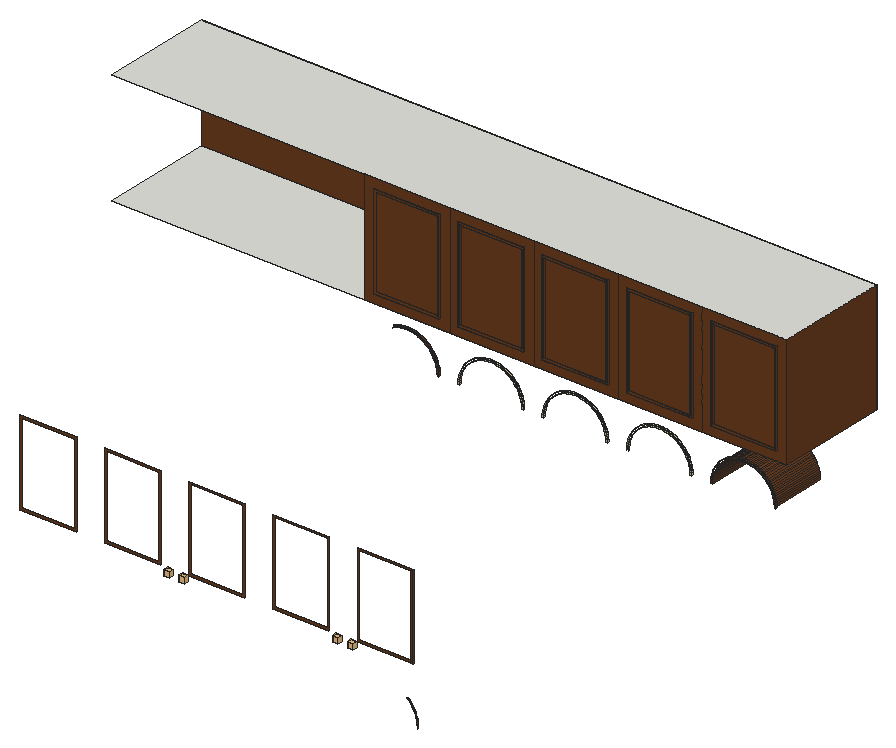
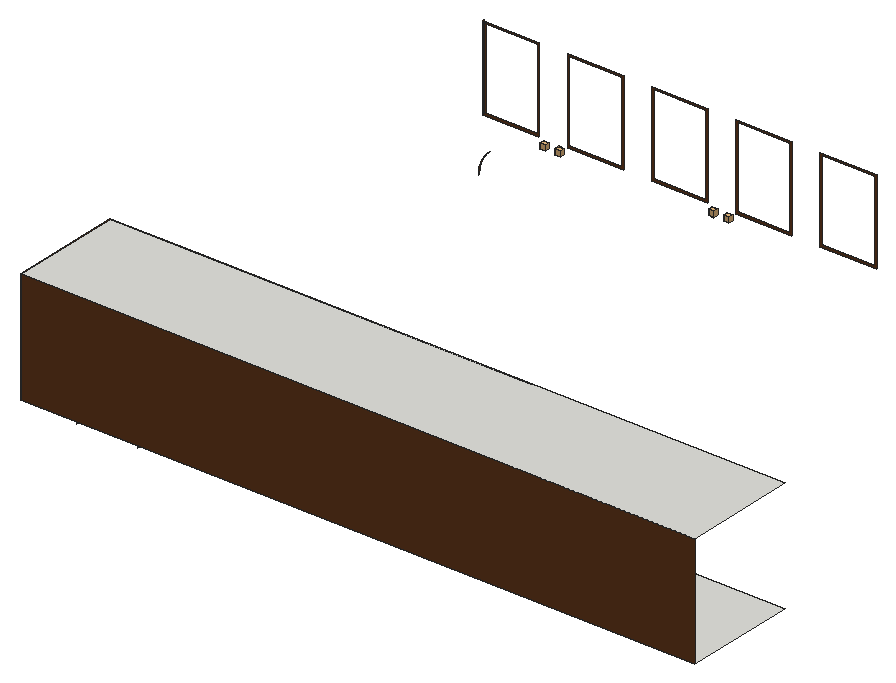
# SketchUp Ruby script. Lengths in inches.
U = 1.inch
M = Sketchup.active_model
def pt(a) = Geom::Point3d.new(a.map { |v| v * U })
def face(e, loops, mat)
  f = e.add_face(loops[0].map { |a| pt(a) })
  loops[1..].each { |l| e.add_face(l.map { |a| pt(a) }).erase! }
  f.material = f.back_material = mat if mat
  f
end
# faces: each face lists its corners as indices into pts; further lists are holes
def faces(e, pts, list, mat = nil) = list.each { |f| face(e, (f[0].is_a?(Array) ? f : [f]).map { |l| l.map { |i| pts[i] } }, mat) }
# xy, xz, yz: faces in a plane at the given z, y or x. An outline is a flat list of corners, or four numbers for a rectangle; further outlines are holes
def ring(l) = l.size == 4 ? [[l[0], l[1]], [l[2], l[1]], [l[2], l[3]], [l[0], l[3]]] : l.each_slice(2).to_a
def flat(e, list, mat, &to3) = list.each { |f| face(e, (f[0].is_a?(Array) ? f : [f]).map { |l| ring(l).map { |u, v| to3.(u, v) } }, mat) }
def xy(e, z, list, mat = nil) = flat(e, list, mat) { |x, y| [x, y, z] }
def xz(e, y, list, mat = nil) = flat(e, list, mat) { |x, z| [x, y, z] }
def yz(e, x, list, mat = nil) = flat(e, list, mat) { |y, z| [x, y, z] }
def lines(e, pts, list) = list.each { |a, b| e.add_line(pt(pts[a]), pt(pts[b])) }
# prism: a flat outline (further loops are holes) pulled along v
def prism(e, loops, v, mat = nil)
  f = face(e, loops, mat); d = Geom::Vector3d.new(v.map { |x| x * U })
  f.pushpull(f.normal.samedirection?(d) ? d.length : -d.length)
end
def box(e, o, s, mat = nil) = prism(e, [[o, [o[0] + s[0], o[1], o[2]], [o[0] + s[0], o[1] + s[1], o[2]], [o[0], o[1] + s[1], o[2]]]], [0, 0, s[2]], mat)
def at(x, y, z, deg = 0) = Geom::Transformation.translation(pt([x, y, z])) * Geom::Transformation.rotation(ORIGIN, Z_AXIS, deg.degrees)
def axes(o, x, y, z) = Geom::Transformation.new([*x, 0, *y, 0, *z, 0, *pt(o).to_a, 1])
def part(name) = M.definitions.add(name)
# library, detail: a bought-in or finely detailed component or shape, given as its bounding box
def library(name, o, s) = part(name).tap { |d| box(d.entities, o, s) }
def detail(e, o, s) = box(e.add_group.entities, o, s)
def put(e, d, t, mat = nil) = e.add_instance(d, t).tap { |i| i.material = mat if mat }
def group(e, t, mat = nil) = e.add_group.tap { |g| g.transformation = t; g.material = mat if mat }.entities
root = M.entities
M.materials.add("138_plaster painted wall texture-seamless").color = [214, 198, 153]
M.materials.add("[Wood Veneer 01]").color = [104, 60, 32]
c1 = library("Group\#17",[0,0,0],[1.625,1.625,1.31])
xy(root,85.6,[[158.82,119.8,159.18,132]],"[Wood Veneer 01]")
xy(root,86,[[158.81,119.8,159.19,120]],"[Wood Veneer 01]")
xy(root,88,[[24,120,168,144]])
xy(root,90,[[80,119.8,94,120],[98,119.8,112,120],[116,119.8,130,120],[134,119.8,148,120],[152,119.8,166,120]],"[Wood Veneer 01]")
xy(root,90.4,[[80.4,119.8,93.6,120],[98.4,119.8,111.6,120],[116.4,119.8,129.6,120],[134.4,119.8,147.6,120],[152.4,119.8,165.6,120]],"[Wood Veneer 01]")
xy(root,109.6,[[80.4,119.8,93.6,120],[98.4,119.8,111.6,120],[116.4,119.8,129.6,120],[134.4,119.8,147.6,120],[152.4,119.8,165.6,120]],"[Wood Veneer 01]")
xy(root,110,[[116,119.8,130,120]])
xy(root,110,[[80,119.8,94,120],[98,119.8,112,120],[134,119.8,148,120],[152,119.8,166,120]],"[Wood Veneer 01]")
xy(root,112,[[24,120,168,144]])
xz(root,24.2,[[[81,91,93,109],[81.4,91.4,92.6,108.6]],[[99,91,111,109],[99.4,91.4,110.6,108.6]],[[117,91,129,109],[117.4,91.4,128.6,108.6]],[[135,91,147,109],[135.4,91.4,146.6,108.6]],[[153,91,165,109],[153.4,91.4,164.6,108.6]]],"[Wood Veneer 01]")
xz(root,119.8,[[[80,90,94,110],[80.4,90.4,93.6,109.6]],[[98,90,112,110],[98.4,90.4,111.6,109.6]],[[116,90,130,110],[116.4,90.4,129.6,109.6]],[[134,90,148,110],[134.4,90.4,147.6,109.6]],[[152,90,166,110],[152.4,90.4,165.6,109.6]]],"[Wood Veneer 01]")
xz(root,120,[[[78,88,96,112],[80,90,94,110]],[[96,88,114,112],[98,90,112,110]],[[114,88,132,112],[116,90,130,110]],[[132,88,150,112],[134,90,148,110]],[[150,88,168,112],[152,90,166,110]],
  [80.4,90.4,93.6,109.6],[98.4,90.4,111.6,109.6],[116.4,90.4,129.6,109.6],[134.4,90.4,147.6,109.6],[152.4,90.4,165.6,109.6]],"[Wood Veneer 01]")
xz(root,144,[[24,88,168,112]],"[Wood Veneer 01]")
yz(root,93.6,[[119.8,90.4,120,109.6]],"[Wood Veneer 01]")
yz(root,94,[[119.8,90,120,110]],"[Wood Veneer 01]")
yz(root,98,[[119.8,90,120,110]],"[Wood Veneer 01]")
yz(root,98.4,[[119.8,90.4,120,109.6]],"[Wood Veneer 01]")
yz(root,111.6,[[119.8,90.4,120,109.6]],"[Wood Veneer 01]")
yz(root,112,[[119.8,90,120,110]],"[Wood Veneer 01]")
yz(root,116,[[119.8,90,120,110]],"[Wood Veneer 01]")
yz(root,116.4,[[119.8,90.4,120,109.6]],"[Wood Veneer 01]")
yz(root,129.6,[[119.8,90.4,120,109.6]],"[Wood Veneer 01]")
yz(root,130,[[119.8,90,120,110]],"[Wood Veneer 01]")
yz(root,134,[[119.8,90,120,110]],"[Wood Veneer 01]")
yz(root,134.4,[[119.8,90.4,120,109.6]],"[Wood Veneer 01]")
yz(root,147.6,[[119.8,90.4,120,109.6]],"[Wood Veneer 01]")
yz(root,148,[[119.8,90,120,110]],"[Wood Veneer 01]")
yz(root,152,[[119.8,90,120,110]],"[Wood Veneer 01]")
yz(root,152.4,[[119.8,90.4,120,109.6]],"[Wood Veneer 01]")
yz(root,164.6,[[24,91.4,24.2,108.6]],"[Wood Veneer 01]")
yz(root,165,[[24,91,24.2,109]],"[Wood Veneer 01]")
yz(root,165.6,[[119.8,90.4,120,109.6]],"[Wood Veneer 01]")
yz(root,166,[[119.8,90,120,110]],"[Wood Veneer 01]")
yz(root,168,[[120,88,144,112]],"[Wood Veneer 01]")
p = [[165.99,24,79.41],[166,24,79],[166,24.2,79],[165.99,24.2,79.41],[93.59,120,79.43],[93.6,120,79],
  [93.6,119.8,79],[93.59,119.8,79.43],[94,120,79],[93.99,120,79.46],[93.99,119.8,79.46],[94,119.8,79],
  [98.01,120,79.46],[98,120,79],[98,119.8,79],[98.01,119.8,79.46],[98.4,120,79],[98.41,120,79.43],
  [98.41,119.8,79.43],[98.4,119.8,79],[111.59,120,79.43],[111.6,120,79],[111.6,119.8,79],[111.59,119.8,79.43],
  [112,120,79],[111.99,120,79.46],[111.99,119.8,79.46],[112,119.8,79],[116.01,120,79.46],[116,120,79],
  [116,119.8,79],[116.01,119.8,79.46],[116.4,120,79],[116.41,120,79.43],[116.41,119.8,79.43],[116.4,119.8,79],
  [129.59,120,79.43],[129.6,120,79],[129.6,119.8,79],[129.59,119.8,79.43],[130,120,79],[129.99,120,79.46],
  [129.99,119.8,79.46],[130,119.8,79],[134.01,120,79.46],[134,120,79],[134,119.8,79],[134.01,119.8,79.46],
  [134.4,120,79],[134.41,120,79.43],[134.41,119.8,79.43],[134.4,119.8,79],[147.59,120,79.43],[147.6,120,79],
  [147.6,119.8,79],[147.59,119.8,79.43],[148,120,79],[147.99,120,79.46],[147.99,119.8,79.46],[148,119.8,79],
  [152.01,120,79.39],[152,120,79],[152,119.8,79],[152.01,119.8,79.39],[152.41,132,79.36],[152.41,119.8,79.36],
  [152.4,119.8,79],[152.4,132,79],[165.6,132,79],[165.6,119.8,79],[165.59,119.8,79.36],[165.59,132,79.36],
  [166,120,79],[165.99,120,79.39],[165.99,119.8,79.39],[166,119.8,79],[165.95,24,79.8125],[165.95,24.2,79.8125],
  [93.54,120,79.86],[93.54,119.8,79.86],[98.46,120,79.86],[98.46,119.8,79.86],[111.54,120,79.86],[111.54,119.8,79.86],
  [116.46,120,79.86],[116.46,119.8,79.86],[129.54,120,79.86],[129.54,119.8,79.86],[134.46,120,79.86],[134.46,119.8,79.86],
  [147.54,120,79.86],[147.54,119.8,79.86],[152.04,120,79.77],[152.04,119.8,79.77],[152.44,132,79.73],[152.44,119.8,79.73],
  [165.56,119.8,79.73],[165.56,132,79.73],[165.96,120,79.77],[165.96,119.8,79.77],[93.94,120,79.91],[93.94,119.8,79.91],
  [98.06,120,79.91],[98.06,119.8,79.91],[111.94,120,79.91],[111.94,119.8,79.91],[116.06,120,79.91],[116.06,119.8,79.91],
  [129.94,120,79.91],[129.94,119.8,79.91],[134.06,120,79.91],[134.06,119.8,79.91],[147.94,120,79.91],[147.94,119.8,79.91],
  [152.49,132,80.09],[152.49,119.8,80.09],[165.51,119.8,80.09],[165.51,132,80.09],[165.89,24,80.22],[165.89,24.2,80.22],
  [152.1,120,80.15],[152.1,119.8,80.15],[165.9,120,80.15],[165.9,119.8,80.15],[93.47,120,80.29],[93.47,119.8,80.29],
  [93.87,120,80.37],[93.87,119.8,80.37],[98.13,120,80.37],[98.13,119.8,80.37],[98.53,120,80.29],[98.53,119.8,80.29],
  [111.47,120,80.29],[111.47,119.8,80.29],[111.87,120,80.37],[111.87,119.8,80.37],[116.13,120,80.37],[116.13,119.8,80.37],
  [116.53,120,80.29],[116.53,119.8,80.29],[129.47,120,80.29],[129.47,119.8,80.29],[129.87,120,80.37],[129.87,119.8,80.37],
  [134.13,120,80.37],[134.13,119.8,80.37],[134.53,120,80.29],[134.53,119.8,80.29],[147.47,120,80.29],[147.47,119.8,80.29],
  [147.87,120,80.37],[147.87,119.8,80.37],[152.56,132,80.44],[152.56,119.8,80.44],[165.44,119.8,80.44],[165.44,132,80.44],
  [165.8125,24,80.61],[165.8125,24.2,80.61],[152.17,120,80.53],[152.17,119.8,80.53],[165.83,120,80.53],[165.83,119.8,80.53],
  [93.375,120,80.71],[93.375,119.8,80.71],[98.625,120,80.71],[98.625,119.8,80.71],[111.375,120,80.71],[111.375,119.8,80.71],
  [116.625,120,80.71],[116.625,119.8,80.71],[129.375,120,80.71],[129.375,119.8,80.71],[134.625,120,80.71],[134.625,119.8,80.71],
  [147.375,120,80.71],[147.375,119.8,80.71],[93.76,120,80.8125],[93.76,119.8,80.8125],[98.24,120,80.8125],[98.24,119.8,80.8125],
  [111.76,120,80.8125],[111.76,119.8,80.8125],[116.24,120,80.8125],[116.24,119.8,80.8125],[129.76,120,80.8125],[129.76,119.8,80.8125],
  [134.24,120,80.8125],[134.24,119.8,80.8125],[147.76,120,80.8125],[147.76,119.8,80.8125],[152.65,132,80.8],[152.65,119.8,80.8],
  [165.35,119.8,80.8],[165.35,132,80.8],[152.26,120,80.9],[152.26,119.8,80.9],[165.74,120,80.9],[165.74,119.8,80.9],
  [165.71,24,81.01],[165.71,24.2,81.01],[93.25,120,81.12],[93.25,119.8,81.12],[98.75,120,81.12],[98.75,119.8,81.12],
  [111.25,120,81.12],[111.25,119.8,81.12],[116.75,120,81.12],[116.75,119.8,81.12],[129.25,120,81.12],[129.25,119.8,81.12],
  [134.75,120,81.12],[134.75,119.8,81.12],[147.25,120,81.12],[147.25,119.8,81.12],[93.63,120,81.25],[93.63,119.8,81.25],
  [98.37,120,81.25],[98.37,119.8,81.25],[111.63,120,81.25],[111.63,119.8,81.25],[116.37,120,81.25],[116.37,119.8,81.25],
  [129.63,120,81.25],[129.63,119.8,81.25],[134.37,120,81.25],[134.37,119.8,81.25],[147.63,120,81.25],[147.63,119.8,81.25],
  [152.76,132,81.14],[152.76,119.8,81.14],[165.24,119.8,81.14],[165.24,132,81.14],[152.38,120,81.27],[152.38,119.8,81.27],
  [165.62,120,81.27],[165.62,119.8,81.27],[165.58,24,81.39],[165.58,24.2,81.39],[93.1,120,81.53],[93.1,119.8,81.53],
  [98.9,120,81.53],[98.9,119.8,81.53],[111.1,120,81.53],[111.1,119.8,81.53],[116.9,120,81.53],[116.9,119.8,81.53],
  [129.1,120,81.53],[129.1,119.8,81.53],[134.9,120,81.53],[134.9,119.8,81.53],[147.1,120,81.53],[147.1,119.8,81.53],
  [152.89,132,81.48],[152.89,119.8,81.48],[165.11,119.8,81.48],[165.11,132,81.48],[93.47,120,81.68],[93.47,119.8,81.68],
  [98.53,120,81.68],[98.53,119.8,81.68],[111.47,120,81.68],[111.47,119.8,81.68],[116.53,120,81.68],[116.53,119.8,81.68],
  [129.47,120,81.68],[129.47,119.8,81.68],[134.53,120,81.68],[134.53,119.8,81.68],[147.47,120,81.68],[147.47,119.8,81.68],
  [152.51,120,81.63],[152.51,119.8,81.63],[165.49,120,81.63],[165.49,119.8,81.63],[165.43,24,81.77],[165.43,24.2,81.77],
  [92.92,120,81.92],[92.92,119.8,81.92],[99.08,120,81.92],[99.08,119.8,81.92],[110.92,120,81.92],[110.92,119.8,81.92],
  [117.08,120,81.92],[117.08,119.8,81.92],[128.92,120,81.92],[128.92,119.8,81.92],[135.08,120,81.92],[135.08,119.8,81.92],
  [146.92,120,81.92],[146.92,119.8,81.92],[153.03,132,81.82],[153.03,119.8,81.82],[164.97,119.8,81.82],[164.97,132,81.82],
  [152.67,120,81.99],[152.67,119.8,81.99],[165.33,120,81.99],[165.33,119.8,81.99],[93.28,120,82.1],[93.28,119.8,82.1],
  [98.72,120,82.1],[98.72,119.8,82.1],[111.28,120,82.1],[111.28,119.8,82.1],[116.72,120,82.1],[116.72,119.8,82.1],
  [129.28,120,82.1],[129.28,119.8,82.1],[134.72,120,82.1],[134.72,119.8,82.1],[147.28,120,82.1],[147.28,119.8,82.1],
  [165.26,24,82.14],[165.26,24.2,82.14],[153.2,132,82.14],[153.2,119.8,82.14],[164.8,119.8,82.14],[164.8,132,82.14],
  [92.72,120,82.3],[92.72,119.8,82.3],[99.28,120,82.3],[99.28,119.8,82.3],[110.72,120,82.3],[110.72,119.8,82.3],
  [117.28,120,82.3],[117.28,119.8,82.3],[128.72,120,82.3],[128.72,119.8,82.3],[135.28,120,82.3],[135.28,119.8,82.3],
  [146.72,120,82.3],[146.72,119.8,82.3],[152.84,120,82.33],[152.84,119.8,82.33],[165.16,120,82.33],[165.16,119.8,82.33],
  [165.0625,24,82.5],[165.0625,24.2,82.5],[93.0625,120,82.5],[93.0625,119.8,82.5],[98.9375,120,82.5],[98.9375,119.8,82.5],
  [111.0625,120,82.5],[111.0625,119.8,82.5],[116.9375,120,82.5],[116.9375,119.8,82.5],[129.0625,120,82.5],[129.0625,119.8,82.5],
  [134.9375,120,82.5],[134.9375,119.8,82.5],[147.0625,120,82.5],[147.0625,119.8,82.5],[153.38,132,82.46],[153.38,119.8,82.46],
  [164.62,119.8,82.46],[164.62,132,82.46],[92.49,120,82.67],[92.49,119.8,82.67],[99.51,120,82.67],[99.51,119.8,82.67],
  [110.49,120,82.67],[110.49,119.8,82.67],[117.51,120,82.67],[117.51,119.8,82.67],[128.49,120,82.67],[128.49,119.8,82.67],
  [135.51,120,82.67],[135.51,119.8,82.67],[146.49,120,82.67],[146.49,119.8,82.67],[153.04,120,82.67],[153.04,119.8,82.67],
  [164.96,120,82.67],[164.96,119.8,82.67],[164.85,24,82.85],[164.85,24.2,82.85],[92.82,120,82.89],[92.82,119.8,82.89],
  [99.18,120,82.89],[99.18,119.8,82.89],[110.82,120,82.89],[110.82,119.8,82.89],[117.18,120,82.89],[117.18,119.8,82.89],
  [128.82,120,82.89],[128.82,119.8,82.89],[135.18,120,82.89],[135.18,119.8,82.89],[146.82,120,82.89],[146.82,119.8,82.89],
  [153.58,132,82.76],[153.58,119.8,82.76],[164.42,119.8,82.76],[164.42,132,82.76],[92.24,120,83.02],[92.24,119.8,83.02],
  [99.76,120,83.02],[99.76,119.8,83.02],[110.24,120,83.02],[110.24,119.8,83.02],[117.76,120,83.02],[117.76,119.8,83.02],
  [128.24,120,83.02],[128.24,119.8,83.02],[135.76,120,83.02],[135.76,119.8,83.02],[146.24,120,83.02],[146.24,119.8,83.02],
  [153.25,120,82.99],[153.25,119.8,82.99],[164.75,120,82.99],[164.75,119.8,82.99],[164.61,24,83.18],[164.61,24.2,83.18],
  [153.79,132,83.05],[153.79,119.8,83.05],[164.21,119.8,83.05],[164.21,132,83.05],[92.55,120,83.26],[92.55,119.8,83.26],
  [99.45,120,83.26],[99.45,119.8,83.26],[110.55,120,83.26],[110.55,119.8,83.26],[117.45,120,83.26],[117.45,119.8,83.26],
  [128.55,120,83.26],[128.55,119.8,83.26],[135.45,120,83.26],[135.45,119.8,83.26],[146.55,120,83.26],[146.55,119.8,83.26],
  [91.96,120,83.35],[91.96,119.8,83.35],[100.04,120,83.35],[100.04,119.8,83.35],[109.96,120,83.35],[109.96,119.8,83.35],
  [118.04,120,83.35],[118.04,119.8,83.35],[127.96,120,83.35],[127.96,119.8,83.35],[136.04,120,83.35],[136.04,119.8,83.35],
  [145.96,120,83.35],[145.96,119.8,83.35],[153.48,120,83.3],[153.48,119.8,83.3],[164.52,120,83.3],[164.52,119.8,83.3],
  [154.02,132,83.33],[154.02,119.8,83.33],[163.98,119.8,83.33],[163.98,132,83.33],[164.36,24,83.5],[164.36,24.2,83.5],
  [92.26,120,83.62],[92.26,119.8,83.62],[99.74,120,83.62],[99.74,119.8,83.62],[110.26,120,83.62],[110.26,119.8,83.62],
  [117.74,120,83.62],[117.74,119.8,83.62],[128.26,120,83.62],[128.26,119.8,83.62],[135.74,120,83.62],[135.74,119.8,83.62],
  [146.26,120,83.62],[146.26,119.8,83.62],[153.72,120,83.6],[153.72,119.8,83.6],[154.27,132,83.6],[154.27,119.8,83.6],
  [163.73,119.8,83.6],[163.73,132,83.6],[164.28,120,83.6],[164.28,119.8,83.6],[91.67,120,83.67],[91.67,119.8,83.67],
  [100.33,120,83.67],[100.33,119.8,83.67],[109.67,120,83.67],[109.67,119.8,83.67],[118.33,120,83.67],[118.33,119.8,83.67],
  [127.67,120,83.67],[127.67,119.8,83.67],[136.33,120,83.67],[136.33,119.8,83.67],[145.67,120,83.67],[145.67,119.8,83.67],
  [164.09,24,83.8],[164.09,24.2,83.8],[91.95,120,83.95],[91.95,119.8,83.95],[100.05,120,83.95],[100.05,119.8,83.95],
  [109.95,120,83.95],[109.95,119.8,83.95],[118.05,120,83.95],[118.05,119.8,83.95],[127.95,120,83.95],[127.95,119.8,83.95],
  [136.05,120,83.95],[136.05,119.8,83.95],[145.95,120,83.95],[145.95,119.8,83.95],[153.98,120,83.88],[153.98,119.8,83.88],
  [154.53,132,83.86],[154.53,119.8,83.86],[163.47,119.8,83.86],[163.47,132,83.86],[164.02,120,83.88],[164.02,119.8,83.88],
  [91.35,120,83.96],[91.35,119.8,83.96],[100.65,120,83.96],[100.65,119.8,83.96],[109.35,120,83.96],[109.35,119.8,83.96],
  [118.65,120,83.96],[118.65,119.8,83.96],[127.35,120,83.96],[127.35,119.8,83.96],[136.65,120,83.96],[136.65,119.8,83.96],
  [145.35,120,83.96],[145.35,119.8,83.96],[163.8,24,84.09],[163.8,24.2,84.09],[91.62,120,84.26],[91.62,119.8,84.26],
  [100.38,120,84.26],[100.38,119.8,84.26],[109.62,120,84.26],[109.62,119.8,84.26],[118.38,120,84.26],[118.38,119.8,84.26],
  [127.62,120,84.26],[127.62,119.8,84.26],[136.38,120,84.26],[136.38,119.8,84.26],[145.62,120,84.26],[145.62,119.8,84.26],
  [154.26,120,84.15],[154.26,119.8,84.15],[154.8,132,84.09],[154.8,119.8,84.09],[163.2,119.8,84.09],[163.2,132,84.09],
  [163.74,120,84.15],[163.74,119.8,84.15],[91.02,120,84.24],[91.02,119.8,84.24],[100.98,120,84.24],[100.98,119.8,84.24],
  [109.02,120,84.24],[109.02,119.8,84.24],[118.98,120,84.24],[118.98,119.8,84.24],[127.02,120,84.24],[127.02,119.8,84.24],
  [136.98,120,84.24],[136.98,119.8,84.24],[145.02,120,84.24],[145.02,119.8,84.24],[155.09,132,84.32],[155.09,119.8,84.32],
  [162.91,119.8,84.32],[162.91,132,84.32],[90.67,120,84.49],[90.67,119.8,84.49],[101.33,120,84.49],[101.33,119.8,84.49],
  [108.67,120,84.49],[108.67,119.8,84.49],[119.33,120,84.49],[119.33,119.8,84.49],[126.67,120,84.49],[126.67,119.8,84.49],
  [137.33,120,84.49],[137.33,119.8,84.49],[144.67,120,84.49],[144.67,119.8,84.49],[154.55,120,84.4],[154.55,119.8,84.4],
  [163.45,120,84.4],[163.45,119.8,84.4],[91.26,120,84.55],[91.26,119.8,84.55],[100.74,120,84.55],[100.74,119.8,84.55],
  [109.26,120,84.55],[109.26,119.8,84.55],[118.74,120,84.55],[118.74,119.8,84.55],[127.26,120,84.55],[127.26,119.8,84.55],
  [136.74,120,84.55],[136.74,119.8,84.55],[145.26,120,84.55],[145.26,119.8,84.55],[155.39,132,84.53],[155.39,119.8,84.53],
  [162.61,119.8,84.53],[162.61,132,84.53],[154.85,120,84.64],[154.85,119.8,84.64],[163.15,120,84.64],[163.15,119.8,84.64],
  [90.3,120,84.72],[90.3,119.8,84.72],[101.7,120,84.72],[101.7,119.8,84.72],[108.3,120,84.72],[108.3,119.8,84.72],
  [119.7,120,84.72],[119.7,119.8,84.72],[126.3,120,84.72],[126.3,119.8,84.72],[137.7,120,84.72],[137.7,119.8,84.72],
  [144.3,120,84.72],[144.3,119.8,84.72],[155.7,132,84.72],[155.7,119.8,84.72],[162.3,119.8,84.72],[162.3,132,84.72],
  [90.89,120,84.82],[90.89,119.8,84.82],[101.11,120,84.82],[101.11,119.8,84.82],[108.89,120,84.82],[108.89,119.8,84.82],
  [119.11,120,84.82],[119.11,119.8,84.82],[126.89,120,84.82],[126.89,119.8,84.82],[137.11,120,84.82],[137.11,119.8,84.82],
  [144.89,120,84.82],[144.89,119.8,84.82],[155.17,120,84.86],[155.17,119.8,84.86],[162.83,120,84.86],[162.83,119.8,84.86],
  [89.92,120,84.92],[89.92,119.8,84.92],[102.08,120,84.92],[102.08,119.8,84.92],[107.92,120,84.92],[107.92,119.8,84.92],
  [120.08,120,84.92],[120.08,119.8,84.92],[125.92,120,84.92],[125.92,119.8,84.92],[138.08,120,84.92],[138.08,119.8,84.92],
  [143.92,120,84.92],[143.92,119.8,84.92],[156.02,132,84.89],[156.02,119.8,84.89],[161.98,119.8,84.89],[161.98,132,84.89],
  [90.5,120,85.0625],[90.5,119.8,85.0625],[101.5,120,85.0625],[101.5,119.8,85.0625],[108.5,120,85.0625],[108.5,119.8,85.0625],
  [119.5,120,85.0625],[119.5,119.8,85.0625],[126.5,120,85.0625],[126.5,119.8,85.0625],[137.5,120,85.0625],[137.5,119.8,85.0625],
  [144.5,120,85.0625],[144.5,119.8,85.0625],[84.08,120,84.92],[84.47,120,85.1],[84.47,119.8,85.1],[84.08,119.8,84.92],
  [89.53,120,85.1],[89.53,119.8,85.1],[102.47,120,85.1],[102.47,119.8,85.1],[107.53,120,85.1],[107.53,119.8,85.1],
  [120.47,120,85.1],[120.47,119.8,85.1],[125.53,120,85.1],[125.53,119.8,85.1],[138.47,120,85.1],[138.47,119.8,85.1],
  [143.53,120,85.1],[143.53,119.8,85.1],[155.5,120,85.0625],[155.5,119.8,85.0625],[156.35,132,85.04],[156.35,119.8,85.04],
  [161.65,119.8,85.04],[161.65,132,85.04],[162.5,120,85.0625],[162.5,119.8,85.0625],[156.6875,132,85.18],[156.6875,119.8,85.18],
  [161.3125,119.8,85.18],[161.3125,132,85.18],[84.88,120,85.25],[84.88,119.8,85.25],[89.12,120,85.25],[89.12,119.8,85.25],
  [90.1,120,85.28],[90.1,119.8,85.28],[101.9,120,85.28],[101.9,119.8,85.28],[102.88,120,85.25],[102.88,119.8,85.25],
  [107.12,120,85.25],[107.12,119.8,85.25],[108.1,120,85.28],[108.1,119.8,85.28],[119.9,120,85.28],[119.9,119.8,85.28],
  [120.88,120,85.25],[120.88,119.8,85.25],[125.12,120,85.25],[125.12,119.8,85.25],[126.1,120,85.28],[126.1,119.8,85.28],
  [137.9,120,85.28],[137.9,119.8,85.28],[138.88,120,85.25],[138.88,119.8,85.25],[143.12,120,85.25],[143.12,119.8,85.25],
  [144.1,120,85.28],[144.1,119.8,85.28],[155.84,120,85.25],[155.84,119.8,85.25],[162.16,120,85.25],[162.16,119.8,85.25],
  [85.29,120,85.375],[85.29,119.8,85.375],[88.71,120,85.375],[88.71,119.8,85.375],[103.29,120,85.375],[103.29,119.8,85.375],
  [106.71,120,85.375],[106.71,119.8,85.375],[121.29,120,85.375],[121.29,119.8,85.375],[124.71,120,85.375],[124.71,119.8,85.375],
  [139.29,120,85.375],[139.29,119.8,85.375],[142.71,120,85.375],[142.71,119.8,85.375],[156.1875,120,85.41],[156.1875,119.8,85.41],
  [157.03,132,85.3],[157.03,119.8,85.3],[160.97,119.8,85.3],[160.97,132,85.3],[161.8125,120,85.41],[161.8125,119.8,85.41],
  [89.68,120,85.47],[89.68,119.8,85.47],[102.32,120,85.47],[102.32,119.8,85.47],[107.68,120,85.47],[107.68,119.8,85.47],
  [120.32,120,85.47],[120.32,119.8,85.47],[125.68,120,85.47],[125.68,119.8,85.47],[138.32,120,85.47],[138.32,119.8,85.47],
  [143.68,120,85.47],[143.68,119.8,85.47],[157.38,132,85.4],[157.38,119.8,85.4],[160.62,119.8,85.4],[160.62,132,85.4],
  [85.71,120,85.47],[85.71,119.8,85.47],[88.29,120,85.47],[88.29,119.8,85.47],[103.71,120,85.47],[103.71,119.8,85.47],
  [106.29,120,85.47],[106.29,119.8,85.47],[121.71,120,85.47],[121.71,119.8,85.47],[124.29,120,85.47],[124.29,119.8,85.47],
  [139.71,120,85.47],[139.71,119.8,85.47],[142.29,120,85.47],[142.29,119.8,85.47],[156.55,120,85.56],[156.55,119.8,85.56],
  [157.73,132,85.48],[157.73,119.8,85.48],[160.27,119.8,85.48],[160.27,132,85.48],[161.45,120,85.56],[161.45,119.8,85.56],
  [84.75,120,85.63],[84.32,120,85.47],[84.32,119.8,85.47],[84.75,119.8,85.63],[86.14,120,85.54],[86.14,119.8,85.54],
  [86.57,120,85.59],[86.57,119.8,85.59],[87.43,120,85.59],[87.86,120,85.54],[87.86,119.8,85.54],[87.43,119.8,85.59],
  [89.25,120,85.63],[89.25,119.8,85.63],[102.75,120,85.63],[102.75,119.8,85.63],[104.14,120,85.54],[104.14,119.8,85.54],
  [104.57,120,85.59],[104.57,119.8,85.59],[105.43,120,85.59],[105.86,120,85.54],[105.86,119.8,85.54],[105.43,119.8,85.59],
  [107.25,120,85.63],[107.25,119.8,85.63],[120.75,120,85.63],[120.75,119.8,85.63],[122.14,120,85.54],[122.14,119.8,85.54],
  [122.57,120,85.59],[122.57,119.8,85.59],[123.43,120,85.59],[123.86,120,85.54],[123.86,119.8,85.54],[123.43,119.8,85.59],
  [125.25,120,85.63],[125.25,119.8,85.63],[138.75,120,85.63],[138.75,119.8,85.63],[140.14,120,85.54],[140.14,119.8,85.54],
  [140.57,120,85.59],[140.57,119.8,85.59],[141.43,120,85.59],[141.86,120,85.54],[141.86,119.8,85.54],[141.43,119.8,85.59],
  [143.25,120,85.63],[143.25,119.8,85.63],[158.09,132,85.54],[158.09,119.8,85.54],[158.45,132,85.58],[158.45,119.8,85.58],
  [159.91,132,85.54],[159.91,119.8,85.54],[159.55,119.8,85.58],[159.55,132,85.58],[85.1875,120,85.76],[85.1875,119.8,85.76],
  [87,120,85.6],[87,119.8,85.6],[88.8125,120,85.76],[88.8125,119.8,85.76],[103.1875,120,85.76],[103.1875,119.8,85.76],
  [105,120,85.6],[105,119.8,85.6],[106.8125,120,85.76],[106.8125,119.8,85.76],[121.1875,120,85.76],[121.1875,119.8,85.76],
  [123,120,85.6],[123,119.8,85.6],[124.8125,120,85.76],[124.8125,119.8,85.76],[139.1875,120,85.76],[139.1875,119.8,85.76],
  [141,120,85.6],[141,119.8,85.6],[142.8125,120,85.76],[142.8125,119.8,85.76],[156.91,120,85.68],[156.91,119.8,85.68],
  [158.82,132,85.6],[158.82,119.8,85.6],[159.18,119.8,85.6],[159.18,132,85.6],[161.09,120,85.68],[161.09,119.8,85.68],
  [157.28,120,85.79],[157.28,119.8,85.79],[160.72,120,85.79],[160.72,119.8,85.79],[85.63,120,85.87],[85.63,119.8,85.87],
  [88.37,120,85.87],[88.37,119.8,85.87],[103.63,120,85.87],[103.63,119.8,85.87],[106.37,120,85.87],[106.37,119.8,85.87],
  [121.63,120,85.87],[121.63,119.8,85.87],[124.37,120,85.87],[124.37,119.8,85.87],[139.63,120,85.87],[139.63,119.8,85.87],
  [142.37,120,85.87],[142.37,119.8,85.87],[157.66,120,85.87],[157.66,119.8,85.87],[160.34,120,85.87],[160.34,119.8,85.87],
  [86.09,120,85.94],[86.09,119.8,85.94],[86.54,120,85.99],[86.54,119.8,85.99],[87.91,120,85.94],[87.46,120,85.99],
  [87.46,119.8,85.99],[87.91,119.8,85.94],[104.09,120,85.94],[104.09,119.8,85.94],[104.54,120,85.99],[104.54,119.8,85.99],
  [105.91,120,85.94],[105.46,120,85.99],[105.46,119.8,85.99],[105.91,119.8,85.94],[122.09,120,85.94],[122.09,119.8,85.94],
  [122.54,120,85.99],[122.54,119.8,85.99],[123.91,120,85.94],[123.46,120,85.99],[123.46,119.8,85.99],[123.91,119.8,85.94],
  [140.09,120,85.94],[140.09,119.8,85.94],[140.54,120,85.99],[140.54,119.8,85.99],[141.91,120,85.94],[141.46,120,85.99],
  [141.46,119.8,85.99],[141.91,119.8,85.94],[158.04,120,85.93],[158.04,119.8,85.93],[158.42,120,85.98],[158.42,119.8,85.98],
  [159.96,120,85.93],[159.58,120,85.98],[159.58,119.8,85.98],[159.96,119.8,85.93],[87,120,86],[87,119.8,86],
  [105,120,86],[105,119.8,86],[123,120,86],[123,119.8,86],[141,120,86],[141,119.8,86],
  [158.81,120,86],[158.81,119.8,86],[159.19,120,86],[159.19,119.8,86]]
faces(root,p,[[0,1,2,3],[4,5,6,7],[8,9,10,11],[60,61,62,63],[64,65,66,67],[68,69,70,71],[72,73,74,75],[76,0,3,77],
  [78,4,7,79],[92,60,63,93],[94,95,65,64],[71,70,96,97],[73,98,99,74],[9,100,101,10],[114,115,95,94],[97,96,116,117],
  [118,76,77,119],[120,92,93,121],[98,122,123,99],[124,78,79,125],[100,126,127,101],[152,153,115,114],[117,116,154,155],[156,118,119,157],
  [158,120,121,159],[122,160,161,123],[162,124,125,163],[126,176,177,127],[190,191,153,152],[155,154,192,193],[194,158,159,195],[160,196,197,161],
  [198,156,157,199],[200,162,163,201],[176,214,215,177],[228,229,191,190],[193,192,230,231],[232,194,195,233],[196,234,235,197],[236,198,199,237],
  [238,200,201,239],[252,253,229,228],[231,230,254,255],[214,256,257,215],[270,232,233,271],[234,272,273,235],[274,236,237,275],[276,238,239,277],
  [290,291,253,252],[255,254,292,293],[294,270,271,295],[272,296,297,273],[256,298,299,257],[312,274,275,313],[314,315,291,290],[293,292,316,317],
  [318,276,277,319],[332,294,295,333],[296,334,335,297],[336,312,313,337],[298,338,339,299],[352,353,315,314],[317,316,354,355],[356,318,319,357],
  [370,332,333,371],[334,372,373,335],[374,336,337,375],[338,376,377,339],[390,391,353,352],[355,354,392,393],[394,356,357,395],[408,370,371,409],
  [372,410,411,373],[412,374,375,413],[414,415,391,390],[393,392,416,417],[376,418,419,377],[432,394,395,433],[446,408,409,447],[410,448,449,411],
  [450,451,415,414],[417,416,452,453],[454,412,413,455],[418,456,457,419],[470,446,447,471],[472,473,451,450],[453,452,474,475],[448,476,477,449],
  [478,432,433,479],[492,454,455,493],[456,494,495,457],[508,470,471,509],[510,511,473,472],[475,474,512,513],[476,514,515,477],[516,478,479,517],
  [530,492,493,531],[494,532,533,495],[546,508,509,547],[548,549,511,510],[513,512,550,551],[514,552,553,515],[554,516,517,555],[568,569,549,548],
  [551,550,570,571],[572,554,555,573],[586,546,547,587],[552,588,589,553],[532,590,591,533],[604,605,569,568],[571,570,606,607],[608,586,587,609],
  [588,610,611,589],[612,572,573,613],[626,627,605,604],[607,606,628,629],[590,630,631,591],[644,608,609,645],[610,646,647,611],[648,612,613,649],
  [662,663,627,626],[629,628,664,665],[630,666,667,631],[680,681,682,683],[684,648,649,685],[698,644,645,699],[700,701,663,662],[665,664,702,703],
  [646,704,705,647],[706,707,701,700],[703,702,708,709],[681,710,711,682],[712,684,685,713],[666,714,715,667],[740,698,699,741],[704,742,743,705],
  [710,744,745,711],[746,712,713,747],[760,740,741,761],[762,763,707,706],[709,708,764,765],[742,766,767,743],[714,768,769,715],[782,783,763,762],
  [765,764,784,785],[744,786,787,745],[788,746,747,789],[802,760,761,803],[804,805,783,782],[785,784,806,807],[766,808,809,767],[810,811,812,813],
  [786,814,815,787],[814,816,817,815],[818,819,820,821],[819,788,789,820],[768,822,823,769],[860,861,805,804],[862,863,861,860],[864,865,866,867],
  [807,806,865,864],[868,810,813,869],[816,870,871,817],[870,818,821,871],[822,872,873,823],[892,802,803,893],[894,895,863,862],[867,866,896,897],
  [808,898,899,809],[900,892,893,901],[898,902,903,899],[904,868,869,905],[872,906,907,873],[920,900,901,921],[902,922,923,903],[924,904,905,925],
  [926,924,925,927],[928,929,930,931],[906,928,931,907],[956,920,921,957],[958,956,957,959],[960,961,962,963],[922,960,963,923],[964,926,927,965],
  [929,964,965,930],[972,958,959,973],[961,974,975,962]],"[Wood Veneer 01]")
faces(root,p,[[12,13,14,15],[16,17,18,19],[20,21,22,23],[24,25,26,27],[28,29,30,31],[32,33,34,35],[36,37,38,39],[40,41,42,43],
  [44,45,46,47],[48,49,50,51],[52,53,54,55],[56,57,58,59],[17,80,81,18],[82,20,23,83],[33,84,85,34],[86,36,39,87],
  [49,88,89,50],[90,52,55,91],[102,12,15,103],[25,104,105,26],[106,28,31,107],[41,108,109,42],[110,44,47,111],[57,112,113,58],
  [128,102,103,129],[80,130,131,81],[132,82,83,133],[104,134,135,105],[136,106,107,137],[84,138,139,85],[140,86,87,141],[108,142,143,109],
  [144,110,111,145],[88,146,147,89],[148,90,91,149],[112,150,151,113],[130,164,165,131],[166,132,133,167],[138,168,169,139],[170,140,141,171],
  [146,172,173,147],[174,148,149,175],[178,128,129,179],[134,180,181,135],[182,136,137,183],[142,184,185,143],[186,144,145,187],[150,188,189,151],
  [164,202,203,165],[204,166,167,205],[168,206,207,169],[208,170,171,209],[172,210,211,173],[212,174,175,213],[216,178,179,217],[180,218,219,181],
  [220,182,183,221],[184,222,223,185],[224,186,187,225],[188,226,227,189],[202,240,241,203],[242,204,205,243],[206,244,245,207],[246,208,209,247],
  [210,248,249,211],[250,212,213,251],[258,216,217,259],[218,260,261,219],[262,220,221,263],[222,264,265,223],[266,224,225,267],[226,268,269,227],
  [240,278,279,241],[280,242,243,281],[244,282,283,245],[284,246,247,285],[248,286,287,249],[288,250,251,289],[300,258,259,301],[260,302,303,261],
  [304,262,263,305],[264,306,307,265],[308,266,267,309],[268,310,311,269],[278,320,321,279],[322,280,281,323],[282,324,325,283],[326,284,285,327],
  [286,328,329,287],[330,288,289,331],[340,300,301,341],[302,342,343,303],[344,304,305,345],[306,346,347,307],[348,308,309,349],[310,350,351,311],
  [320,358,359,321],[360,322,323,361],[324,362,363,325],[364,326,327,365],[328,366,367,329],[368,330,331,369],[378,340,341,379],[342,380,381,343],
  [382,344,345,383],[346,384,385,347],[386,348,349,387],[350,388,389,351],[358,396,397,359],[398,360,361,399],[362,400,401,363],[402,364,365,403],
  [366,404,405,367],[406,368,369,407],[420,378,379,421],[380,422,423,381],[424,382,383,425],[384,426,427,385],[428,386,387,429],[388,430,431,389],
  [396,434,435,397],[436,398,399,437],[400,438,439,401],[440,402,403,441],[404,442,443,405],[444,406,407,445],[458,420,421,459],[422,460,461,423],
  [462,424,425,463],[426,464,465,427],[466,428,429,467],[430,468,469,431],[434,480,481,435],[482,436,437,483],[438,484,485,439],[486,440,441,487],
  [442,488,489,443],[490,444,445,491],[496,458,459,497],[460,498,499,461],[500,462,463,501],[464,502,503,465],[504,466,467,505],[468,506,507,469],
  [480,518,519,481],[520,482,483,521],[484,522,523,485],[524,486,487,525],[488,526,527,489],[528,490,491,529],[534,496,497,535],[498,536,537,499],
  [538,500,501,539],[502,540,541,503],[542,504,505,543],[506,544,545,507],[518,556,557,519],[558,520,521,559],[522,560,561,523],[562,524,525,563],
  [526,564,565,527],[566,528,529,567],[556,574,575,557],[576,558,559,577],[560,578,579,561],[580,562,563,581],[564,582,583,565],[584,566,567,585],
  [592,534,535,593],[536,594,595,537],[596,538,539,597],[540,598,599,541],[600,542,543,601],[544,602,603,545],[574,614,615,575],[616,576,577,617],
  [578,618,619,579],[620,580,581,621],[582,622,623,583],[624,584,585,625],[632,592,593,633],[594,634,635,595],[636,596,597,637],[598,638,639,599],
  [640,600,601,641],[602,642,643,603],[614,650,651,615],[652,616,617,653],[618,654,655,619],[656,620,621,657],[622,658,659,623],[660,624,625,661],
  [668,632,633,669],[634,670,671,635],[672,636,637,673],[638,674,675,639],[676,640,641,677],[642,678,679,643],[650,686,687,651],[688,652,653,689],
  [654,690,691,655],[692,656,657,693],[658,694,695,659],[696,660,661,697],[716,668,669,717],[686,718,719,687],[720,688,689,721],[670,722,723,671],
  [724,672,673,725],[690,726,727,691],[728,692,693,729],[674,730,731,675],[732,676,677,733],[694,734,735,695],[736,696,697,737],[678,738,739,679],
  [718,748,749,719],[750,720,721,751],[726,752,753,727],[754,728,729,755],[734,756,757,735],[758,736,737,759],[770,716,717,771],[722,772,773,723],
  [774,724,725,775],[730,776,777,731],[778,732,733,779],[738,780,781,739],[748,790,791,749],[792,750,751,793],[752,794,795,753],[796,754,755,797],
  [756,798,799,757],[800,758,759,801],[824,770,771,825],[790,826,827,791],[826,828,829,827],[830,831,832,833],[831,792,793,832],[772,834,835,773],
  [836,774,775,837],[794,838,839,795],[838,840,841,839],[842,843,844,845],[843,796,797,844],[776,846,847,777],[848,778,779,849],[798,850,851,799],
  [850,852,853,851],[854,855,856,857],[855,800,801,856],[780,858,859,781],[874,824,825,875],[828,876,877,829],[876,830,833,877],[834,878,879,835],
  [880,836,837,881],[840,882,883,841],[882,842,845,883],[846,884,885,847],[886,848,849,887],[852,888,889,853],[888,854,857,889],[858,890,891,859],
  [908,874,875,909],[878,910,911,879],[912,880,881,913],[884,914,915,885],[916,886,887,917],[890,918,919,891],[932,908,909,933],[934,932,933,935],
  [936,937,938,939],[910,936,939,911],[940,912,913,941],[942,940,941,943],[944,945,946,947],[914,944,947,915],[948,916,917,949],[950,948,949,951],
  [952,953,954,955],[918,952,955,919],[966,934,935,967],[937,966,967,938],[968,942,943,969],[945,968,969,946],[970,950,951,971],[953,970,971,954]],"138_plaster painted wall texture-seamless")
put(root,c1,axes([111.83,24,90.42],[0.75,0,0],[0,0,-0.75],[0,0.75,0]),"[Wood Veneer 01]")
put(root,c1,axes([115.02,24,90.42],[0.75,0,0],[0,0,-0.75],[0,0.75,0]),"[Wood Veneer 01]")
put(root,c1,axes([147.83,24,90.42],[0.75,0,0],[0,0,-0.75],[0,0.75,0]),"[Wood Veneer 01]")
put(root,c1,axes([151.02,24,90.42],[0.75,0,0],[0,0,-0.75],[0,0.75,0]),"[Wood Veneer 01]")
